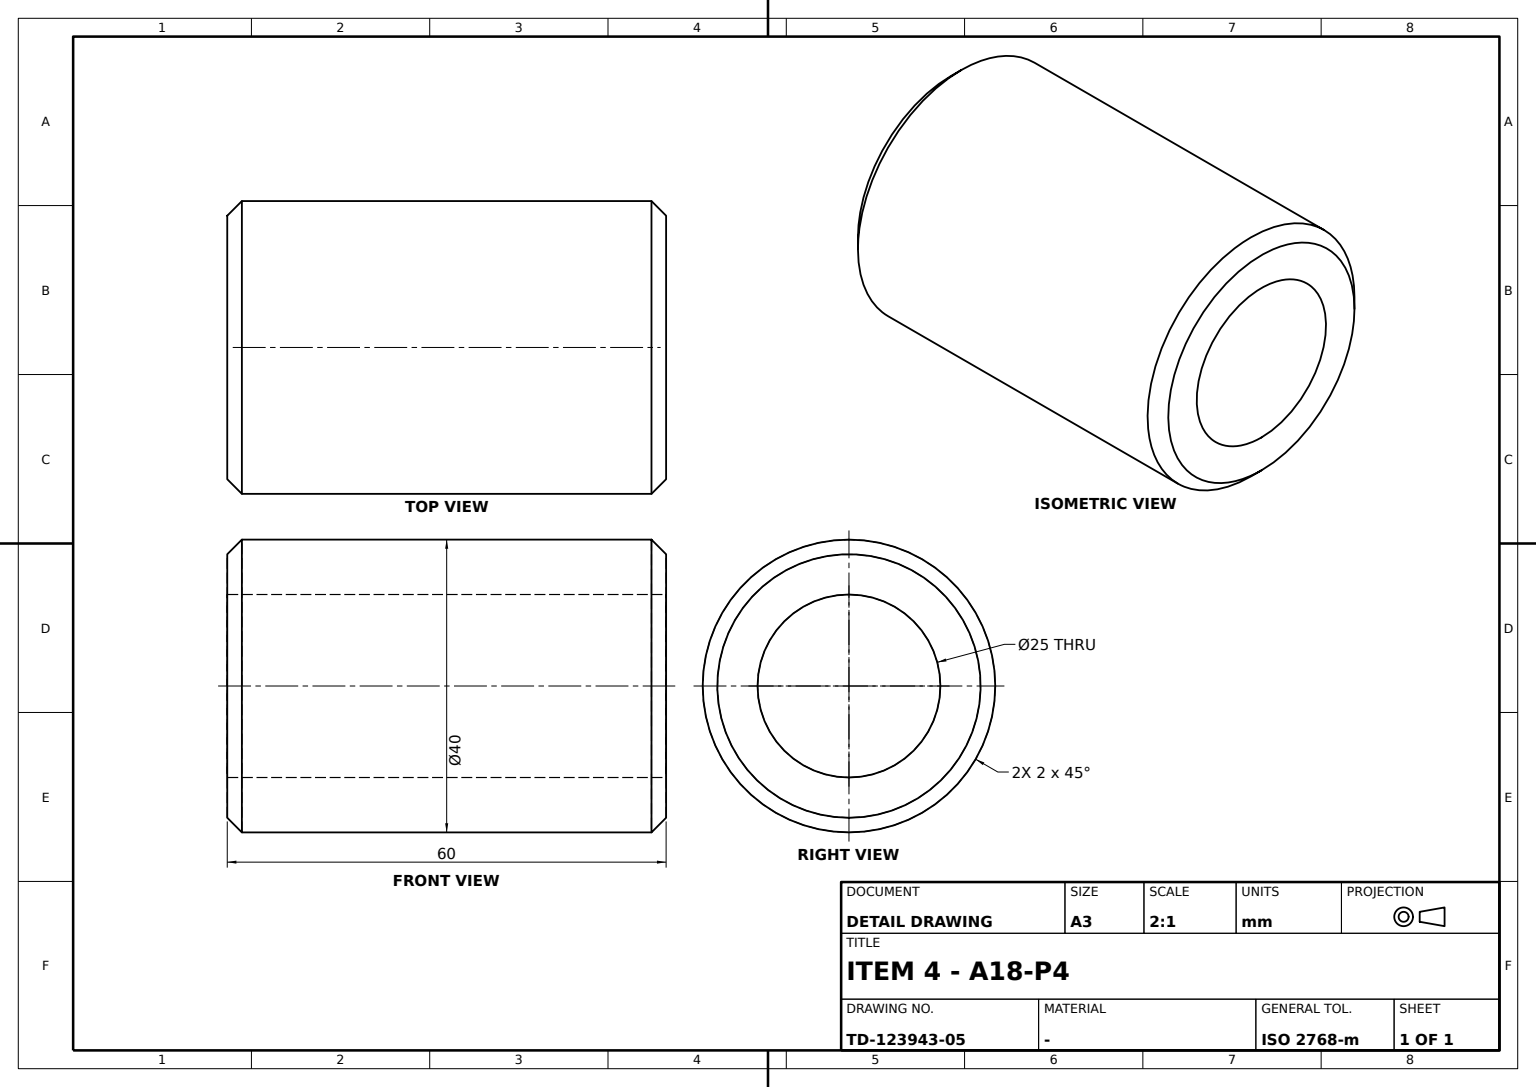
ISO-10303-21;
HEADER;
FILE_DESCRIPTION((''),'2;1');
FILE_NAME('','',(''),(''),'','','');
FILE_SCHEMA(('AUTOMOTIVE_DESIGN'));
ENDSEC;
DATA;
#1=APPLICATION_CONTEXT('');
#2=PRODUCT_CONTEXT('',#1,'mechanical');
#3=PRODUCT('','','',(#2));
#4=PRODUCT_DEFINITION_FORMATION('','',#3);
#5=PRODUCT_DEFINITION_CONTEXT('',#1,'design');
#6=PRODUCT_DEFINITION('','',#4,#5);
#7=PRODUCT_DEFINITION_SHAPE('','',#6);
#8=(LENGTH_UNIT()NAMED_UNIT(*)SI_UNIT(.MILLI.,.METRE.));
#9=(NAMED_UNIT(*)PLANE_ANGLE_UNIT()SI_UNIT($,.RADIAN.));
#10=(NAMED_UNIT(*)SI_UNIT($,.STERADIAN.)SOLID_ANGLE_UNIT());
#11=UNCERTAINTY_MEASURE_WITH_UNIT(LENGTH_MEASURE(0.005),#8,'distance_accuracy_value','');
#12=(GEOMETRIC_REPRESENTATION_CONTEXT(3)GLOBAL_UNCERTAINTY_ASSIGNED_CONTEXT((#11))GLOBAL_UNIT_ASSIGNED_CONTEXT((#8,#9,#10))REPRESENTATION_CONTEXT('',''));
#13=CARTESIAN_POINT('',(12.5,0.,0.));
#14=VERTEX_POINT('',#13);
#15=CARTESIAN_POINT('',(0.,0.,0.));
#16=DIRECTION('',(0.,0.,1.));
#17=DIRECTION('',(1.,0.,0.));
#18=AXIS2_PLACEMENT_3D('',#15,#16,#17);
#19=CIRCLE('',#18,12.5);
#20=EDGE_CURVE('',#14,#14,#19,.T.);
#21=ORIENTED_EDGE('',*,*,#20,.T.);
#22=EDGE_LOOP('',(#21));
#23=FACE_BOUND('',#22,.T.);
#24=CARTESIAN_POINT('',(18.,0.,0.));
#25=VERTEX_POINT('',#24);
#26=CIRCLE('',#18,18.);
#27=EDGE_CURVE('',#25,#25,#26,.T.);
#28=ORIENTED_EDGE('',*,*,#27,.F.);
#29=EDGE_LOOP('',(#28));
#30=FACE_BOUND('',#29,.T.);
#31=DIRECTION('',(0.,1.,0.));
#32=AXIS2_PLACEMENT_3D('',#15,#16,#31);
#33=PLANE('',#32);
#34=ADVANCED_FACE('',(#23,#30),#33,.F.);
#35=CARTESIAN_POINT('',(20.,0.,2.));
#36=VERTEX_POINT('',#35);
#37=CARTESIAN_POINT('',(0.,0.,2.));
#38=AXIS2_PLACEMENT_3D('',#37,#16,#17);
#39=CIRCLE('',#38,20.);
#40=EDGE_CURVE('',#36,#36,#39,.T.);
#41=ORIENTED_EDGE('',*,*,#40,.T.);
#42=EDGE_LOOP('',(#41));
#43=FACE_BOUND('',#42,.T.);
#44=CARTESIAN_POINT('',(-20.,0.,58.));
#45=VERTEX_POINT('',#44);
#46=CARTESIAN_POINT('',(0.,0.,58.));
#47=DIRECTION('',(0.,0.,-1.));
#48=DIRECTION('',(-1.,0.,0.));
#49=AXIS2_PLACEMENT_3D('',#46,#47,#48);
#50=CIRCLE('',#49,20.);
#51=EDGE_CURVE('',#45,#45,#50,.F.);
#52=ORIENTED_EDGE('',*,*,#51,.F.);
#53=EDGE_LOOP('',(#52));
#54=FACE_BOUND('',#53,.T.);
#55=CARTESIAN_POINT('',(0.,0.,30.));
#56=AXIS2_PLACEMENT_3D('',#55,#16,#31);
#57=CYLINDRICAL_SURFACE('',#56,20.);
#58=ADVANCED_FACE('',(#43,#54),#57,.T.);
#59=ORIENTED_EDGE('',*,*,#27,.T.);
#60=EDGE_LOOP('',(#59));
#61=FACE_BOUND('',#60,.T.);
#62=ORIENTED_EDGE('',*,*,#40,.F.);
#63=EDGE_LOOP('',(#62));
#64=FACE_BOUND('',#63,.T.);
#65=CARTESIAN_POINT('',(0.,0.,-18.));
#66=DIRECTION('',(-0.866025404,-0.5,0.));
#67=AXIS2_PLACEMENT_3D('',#65,#16,#66);
#68=CONICAL_SURFACE('',#67,0.,0.785398163);
#69=ADVANCED_FACE('',(#61,#64),#68,.T.);
#70=ORIENTED_EDGE('',*,*,#51,.T.);
#71=EDGE_LOOP('',(#70));
#72=FACE_BOUND('',#71,.T.);
#73=CARTESIAN_POINT('',(18.,0.,60.));
#74=VERTEX_POINT('',#73);
#75=CARTESIAN_POINT('',(0.,0.,60.));
#76=AXIS2_PLACEMENT_3D('',#75,#16,#17);
#77=CIRCLE('',#76,18.);
#78=EDGE_CURVE('',#74,#74,#77,.T.);
#79=ORIENTED_EDGE('',*,*,#78,.F.);
#80=EDGE_LOOP('',(#79));
#81=FACE_BOUND('',#80,.T.);
#82=CARTESIAN_POINT('',(0.,0.,78.));
#83=DIRECTION('',(0.866025404,0.5,0.));
#84=AXIS2_PLACEMENT_3D('',#82,#47,#83);
#85=CONICAL_SURFACE('',#84,0.,0.785398163);
#86=ADVANCED_FACE('',(#72,#81),#85,.T.);
#87=ORIENTED_EDGE('',*,*,#78,.T.);
#88=EDGE_LOOP('',(#87));
#89=FACE_BOUND('',#88,.T.);
#90=CARTESIAN_POINT('',(12.5,0.,60.));
#91=VERTEX_POINT('',#90);
#92=CIRCLE('',#76,12.5);
#93=EDGE_CURVE('',#91,#91,#92,.T.);
#94=ORIENTED_EDGE('',*,*,#93,.F.);
#95=EDGE_LOOP('',(#94));
#96=FACE_BOUND('',#95,.T.);
#97=AXIS2_PLACEMENT_3D('',#75,#16,#31);
#98=PLANE('',#97);
#99=ADVANCED_FACE('',(#89,#96),#98,.T.);
#100=ORIENTED_EDGE('',*,*,#20,.F.);
#101=EDGE_LOOP('',(#100));
#102=FACE_BOUND('',#101,.T.);
#103=ORIENTED_EDGE('',*,*,#93,.T.);
#104=EDGE_LOOP('',(#103));
#105=FACE_BOUND('',#104,.T.);
#106=CYLINDRICAL_SURFACE('',#56,12.5);
#107=ADVANCED_FACE('',(#102,#105),#106,.F.);
#108=CLOSED_SHELL('',(#34,#58,#69,#86,#99,#107));
#109=MANIFOLD_SOLID_BREP('',#108);
#110=ADVANCED_BREP_SHAPE_REPRESENTATION('',(#109),#12);
#111=SHAPE_DEFINITION_REPRESENTATION(#7,#110);
ENDSEC;
END-ISO-10303-21;
